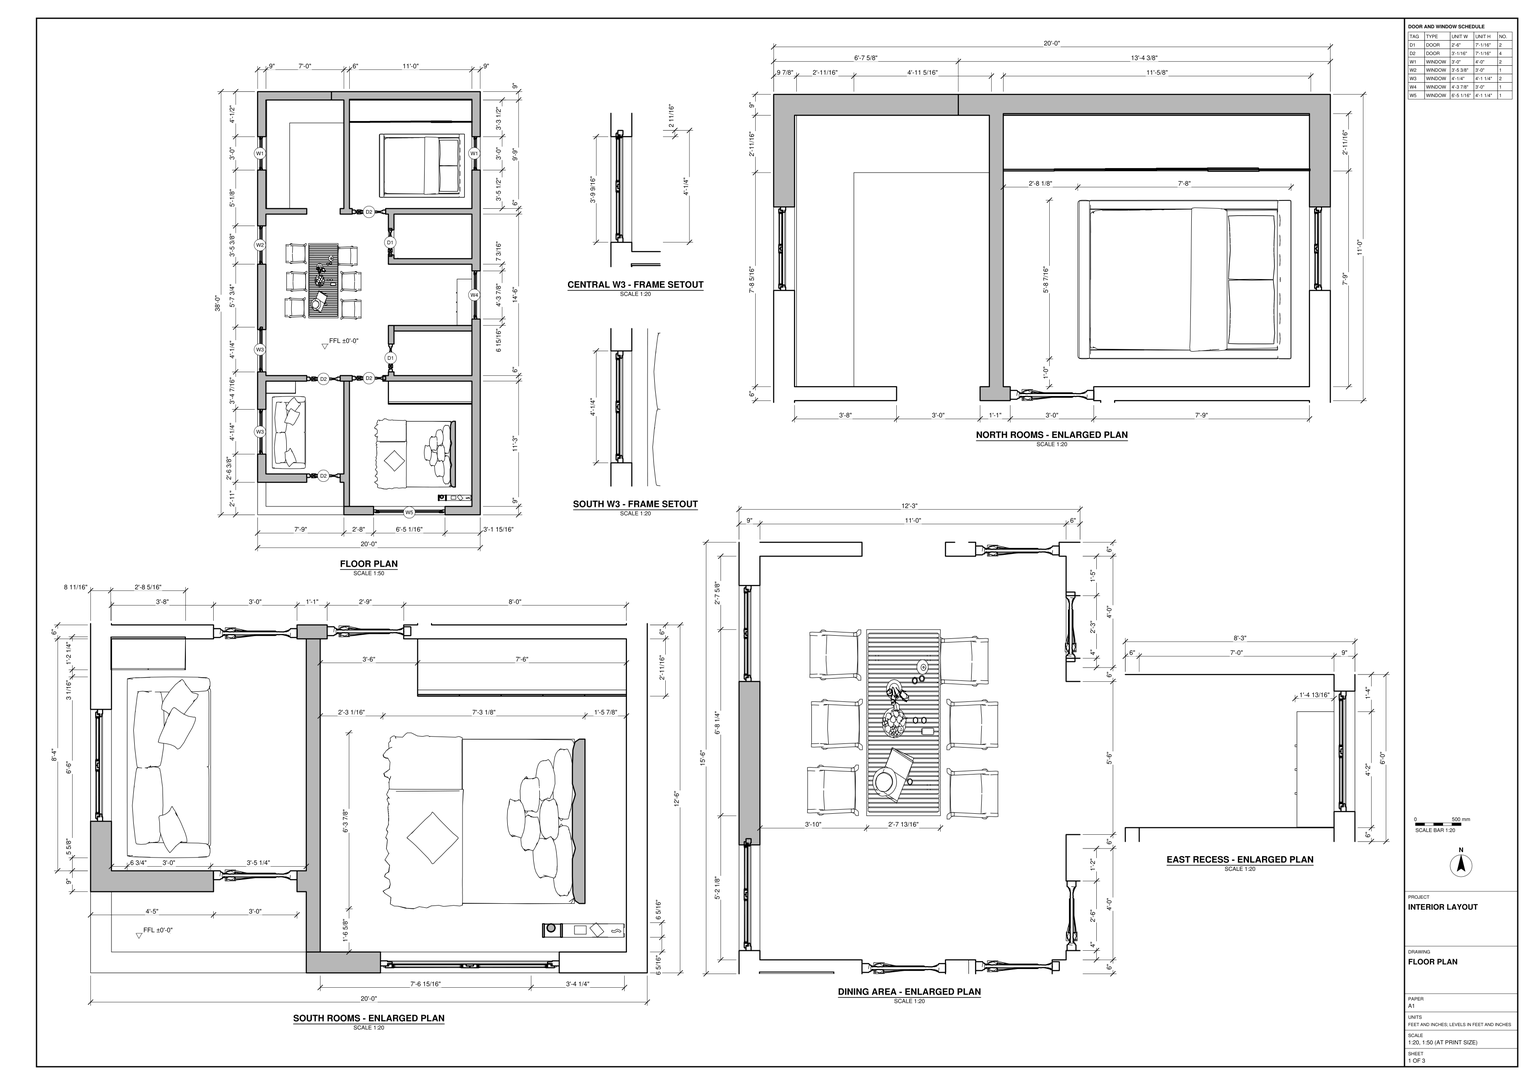
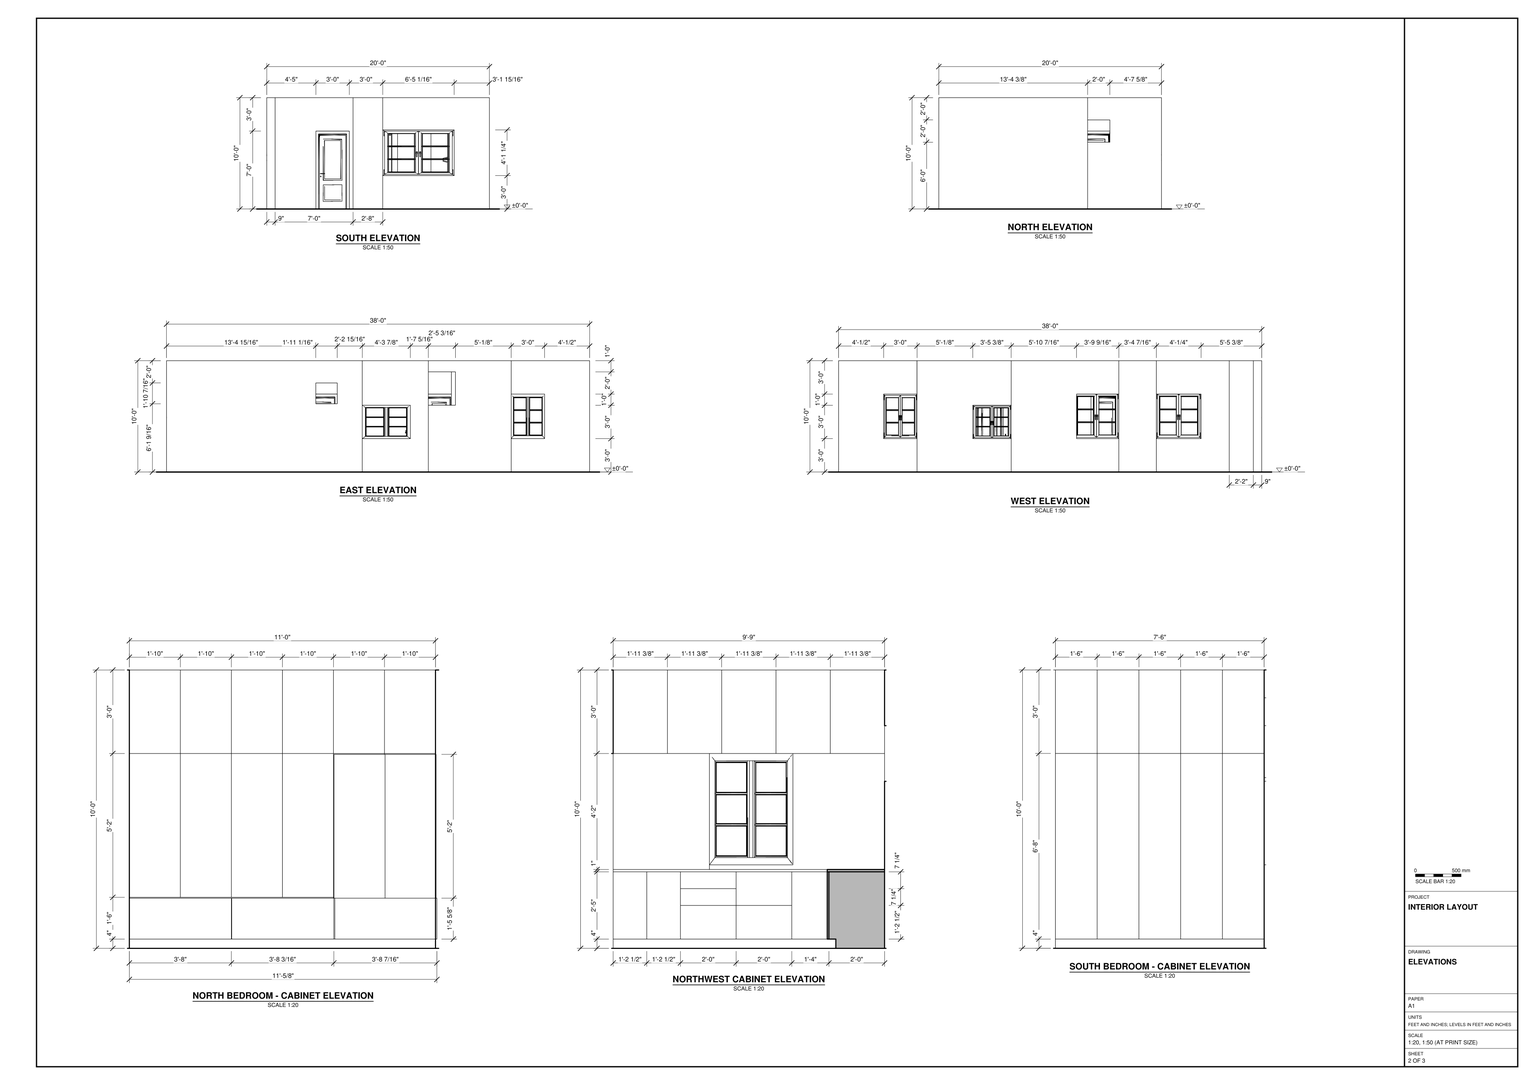
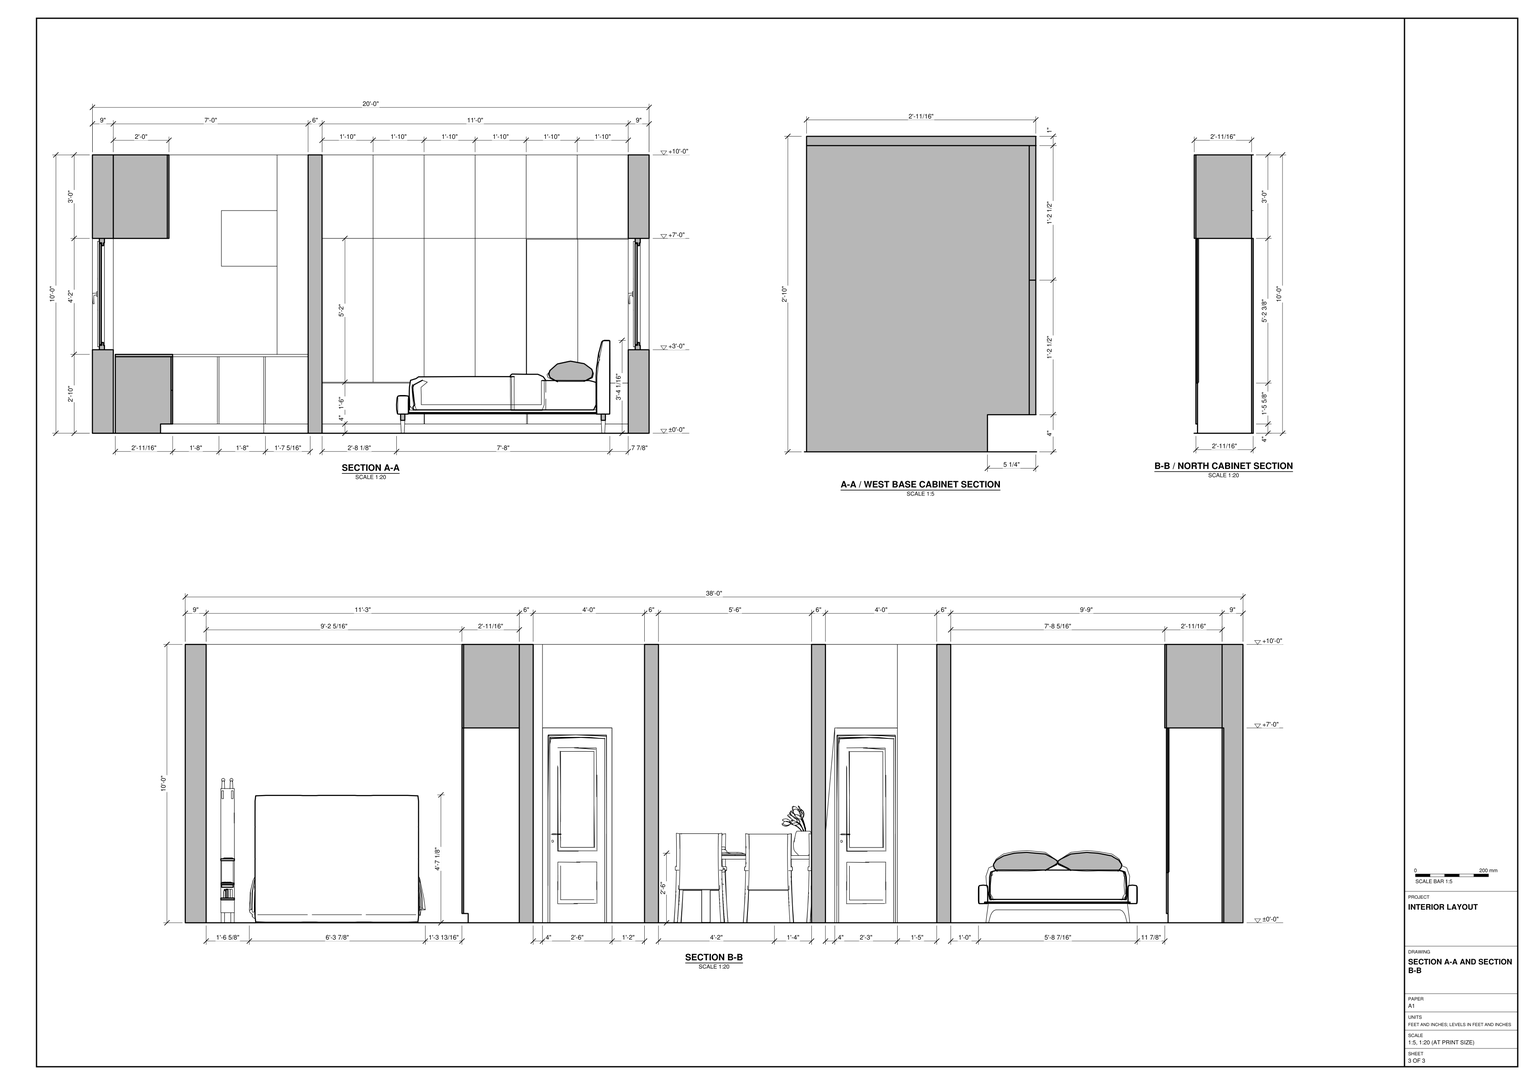
Build the interior in SketchUp from task_files/diagram_01.pdf. Work in feet and inches. The overall model extents are 54'-9 9/16" along X, 65'-5/8" along Y and 10'-13/16" along Z. Use the single finished floor level of ±0'-0". For the room shell itself, follow the 20'-0" by 38'-0" plan and the 10'-0" wall height shown in the sections.

Model the floor slab, the 9" perimeter walls and the 6" partitions, including the setback at the southwest entrance. Lay out the central dining area with its east recess between two enclosed spaces. Use the enlarged plans to position the doors and window units, and the elevations and frame details to set the window heads, sills and divisions.

Place the platform bed in the northeast bedroom, the other bed in the southeast bedroom and the sofa along the west wall of the southwest room. Set the dining table lengthwise with chairs on both long sides. Model the bedroom cabinet runs and the northwest cabinetry around the window, using the cabinet elevations and sections for panel divisions, base units and upper storage. Decor and loose items may be represented by any suitable library components.

Keep shell elements and each furniture or joinery piece in separate groups or components, and use components for repeated parts. Save one SketchUp model as output_files/furnished_two_bedroom_interior_with_built_in_cabinetry.skp.

# SketchUp Ruby script. Lengths in inches.
U = 1.inch
M = Sketchup.active_model
def pt(a) = Geom::Point3d.new(a.map { |v| v * U })
def face(e, loops, mat)
  f = e.add_face(loops[0].map { |a| pt(a) })
  loops[1..].each { |l| e.add_face(l.map { |a| pt(a) }).erase! }
  f.material = f.back_material = mat if mat
  f
end
# faces: each face lists its corners as indices into pts; further lists are holes
def faces(e, pts, list, mat = nil) = list.each { |f| face(e, (f[0].is_a?(Array) ? f : [f]).map { |l| l.map { |i| pts[i] } }, mat) }
# xy, xz, yz: faces in a plane at the given z, y or x. An outline is a flat list of corners, or four numbers for a rectangle; further outlines are holes
def ring(l) = l.size == 4 ? [[l[0], l[1]], [l[2], l[1]], [l[2], l[3]], [l[0], l[3]]] : l.each_slice(2).to_a
def flat(e, list, mat, &to3) = list.each { |f| face(e, (f[0].is_a?(Array) ? f : [f]).map { |l| ring(l).map { |u, v| to3.(u, v) } }, mat) }
def xy(e, z, list, mat = nil) = flat(e, list, mat) { |x, y| [x, y, z] }
def xz(e, y, list, mat = nil) = flat(e, list, mat) { |x, z| [x, y, z] }
def yz(e, x, list, mat = nil) = flat(e, list, mat) { |y, z| [x, y, z] }
def lines(e, pts, list) = list.each { |a, b| e.add_line(pt(pts[a]), pt(pts[b])) }
# prism: a flat outline (further loops are holes) pulled along v
def prism(e, loops, v, mat = nil)
  f = face(e, loops, mat); d = Geom::Vector3d.new(v.map { |x| x * U })
  f.pushpull(f.normal.samedirection?(d) ? d.length : -d.length)
end
def box(e, o, s, mat = nil) = prism(e, [[o, [o[0] + s[0], o[1], o[2]], [o[0] + s[0], o[1] + s[1], o[2]], [o[0], o[1] + s[1], o[2]]]], [0, 0, s[2]], mat)
def at(x, y, z, deg = 0) = Geom::Transformation.translation(pt([x, y, z])) * Geom::Transformation.rotation(ORIGIN, Z_AXIS, deg.degrees)
def axes(o, x, y, z) = Geom::Transformation.new([*x, 0, *y, 0, *z, 0, *pt(o).to_a, 1])
def part(name) = M.definitions.add(name)
# library, detail: a bought-in or finely detailed component or shape, given as its bounding box
def library(name, o, s) = part(name).tap { |d| box(d.entities, o, s) }
def detail(e, o, s) = box(e.add_group.entities, o, s)
def put(e, d, t, mat = nil) = e.add_instance(d, t).tap { |i| i.material = mat if mat }
def group(e, t, mat = nil) = e.add_group.tap { |g| g.transformation = t; g.material = mat if mat }.entities
root = M.entities
M.materials.add("[Basic Tile]").color = [203, 206, 202]
M.materials.add("[Carrera Marble]").color = [207, 207, 207]
M.materials.add("[Color M02]").color = [198, 198, 198]
M.materials.add("[Marble Carrara Gold Floor Tile]").color = [225, 223, 217]
M.materials.add("[Stone Marble]").color = [143, 138, 136]
M.materials.add("[Stone Vein Gray]").color = [166, 165, 165]
M.materials.add("[Wood Bamboo]").color = [177, 105, 43]
M.materials.add("[Wood Board Cork]").color = [215, 201, 115]
M.materials.add("[Wood Lumber ButtJoined]").color = [164, 152, 112]
c1 = library("Tyler Platform Bed",[-34.22,-45.98,0],[68.44,91.98,40.05])
c2 = library("Bed 003",[-38.05,-87.1,0],[75.86,87.1,55.12])
c3 = library("Door 243 074",[-20.11,-2.41,0],[40.22,4.82,86.63])
c4 = library("Dresser 007",[-25,-8.85,0],[50,16.83,30])
c5 = library("Furniture Set 193 001",[-52.77,-40.82,-0.19],[105.38,81.69,50.41])
c6 = library("Giraffe Shelf 96-02",[-20.14,-3.15,0.05],[40.26,6.32,62.23])
c7 = library("Sofa Two-Seater 002",[-38.93,-17.99,0],[77.99,35.98,35.98])
c8 = library("Dresser 002",[-16.14,-8.46,0],[32.28,16.53,40.55])
c9 = library("Window 46-30",[-29.96,-2.6,0],[59.92,5.19,59.84])
c10 = part("Group\#2")
xy(c10.entities,0,[[0,0,22,0.71]])
xy(c10.entities,62,[[0,0,22,0.71]])
xz(c10.entities,0,[[0,0,22,62]],"[Wood Lumber ButtJoined]")
xz(c10.entities,0.71,[[0,0,22,62]])
yz(c10.entities,0,[[0,0,0.71,62]])
yz(c10.entities,22,[[0,0,0.71,62]])
c11 = part("Group\#14")
box(c11.entities,[0,0,0],[22,0.71,62])
c12 = part("Group\#4")
box(c12.entities,[0,0,0],[22,0.71,36])
c13 = part("Group\#9")
box(c13.entities,[0,0,0],[18,0.71,36])
c14 = part("Group\#8")
box(c14.entities,[0,0,0],[18,0.71,80])
c15 = part("Group\#19")
box(c15.entities,[0,-8,0],[0.71,24,14.5])
c16 = part("Group\#17")
box(c16.entities,[0,-8,0],[0.71,24,7.25])
c17 = part("Group\#16")
box(c17.entities,[0.71,0,0],[19.29,0.71,29])
c18 = part("Group\#18")
prism(c18.entities,[[[0,1.5,0],[0,1.5,14.5],[0,1.5,29],[0,16,29],[0,16,0]]],[0.71,0,0])
c19 = part("Group\#22")
box(c19.entities,[0,0,0],[0.71,23.4,36])
xy(root,0,[[[0,0,657.5625,780.625],[20.875,36.8125,260.875,492.8125]],[20.875,36.8125,113.875,36.8125,113.875,45.8125,29.875,45.8125,29.875,71.8125,20.875,71.8125],[113.875,36.8125,145.86,45.8125],[145.86,36.8125,260.875,36.8125,260.875,408.3125,251.875,408.3125,251.875,366.8125,158.875,366.8125,158.875,360.8125,161.875,360.8125,161.875,343.8125,167.875,343.8125,167.875,360.8125,251.875,360.8125,251.875,312.8125,167.875,312.8125,167.875,316.8125,161.875,316.8125,161.875,306.8125,251.875,306.8125,251.875,186.8125,167.875,186.8125,167.875,190.8125,161.875,190.8125,161.875,186.8125,155.875,186.8125,155.875,180.8125,251.875,180.8125,251.875,45.8125,145.86,45.8125],[20.875,71.8125,73.875,71.8125,73.875,80.8125,29.875,80.8125,29.875,180.8125,73.875,180.8125,73.875,186.8125,29.875,186.8125,29.875,360.8125,73.875,360.8125,73.875,366.8125,29.875,366.8125,29.875,483.8125,100.49,483.8125,100.49,492.8125,20.875,492.8125],
  [161.875,156.8125,251.875,180.8125],[109.875,180.8125,119.875,186.8125],[161.875,220.8125,167.875,240.8125],[167.875,234.8125,251.875,240.8125],[161.875,316.8125,167.875,343.8125],
  [109.875,360.8125,122.875,360.8125,122.875,366.8125,119.875,366.8125,119.875,483.8125,251.875,483.8125,251.875,444.3125,260.875,444.3125,260.875,492.8125,100.49,492.8125,100.49,483.8125,113.875,483.8125,113.875,366.8125,109.875,366.8125],[29.875,366.8125,53.875,366.8125,53.875,459.8125,113.875,459.8125,113.875,483.8125,29.875,483.8125],[251.875,408.3125,260.875,444.3125],[119.875,459.8125,251.875,483.8125]])
xy(root,0,[[167.875,312.8125,251.875,360.8125]],"[Stone Marble]")
xy(root,0,[[29.875,45.8125,113.875,45.8125,113.875,71.8125,109.875,71.8125,109.875,80.8125,113.875,80.8125,113.875,180.8125,109.875,180.8125,109.875,186.8125,122.875,186.8125,122.875,180.8125,119.875,180.8125,119.875,45.8125,251.875,45.8125,251.875,156.8125,161.875,156.8125,161.875,180.8125,155.875,180.8125,155.875,186.8125,161.875,186.8125,161.875,190.8125,167.875,190.8125,167.875,186.8125,251.875,186.8125,251.875,234.8125,167.875,234.8125,167.875,220.8125,161.875,220.8125,161.875,240.8125,251.875,240.8125,251.875,306.8125,161.875,306.8125,161.875,360.8125,158.875,360.8125,158.875,366.8125,251.875,366.8125,251.875,459.8125,119.875,459.8125,119.875,366.8125,122.875,366.8125,122.875,360.8125,109.875,360.8125,109.875,366.8125,113.875,366.8125,113.875,459.8125,53.875,459.8125,53.875,366.8125,73.875,366.8125,73.875,360.8125,29.875,360.8125,29.875,186.8125,73.875,186.8125,73.875,180.8125,29.875,180.8125,29.875,80.8125,73.875,80.8125,73.875,71.8125,29.875,71.8125]],"[Stone Vein Gray]")
xy(root,36,[[145.86,36.8125,222.92,45.8125],[20.875,102.16,29.875,150.4],[20.875,190.8125,29.875,236.375],[251.875,247.74,260.875,299.65],[20.875,306.8125,29.875,348.1875],
  [20.875,408.3125,29.875,444.3125]])
xy(root,72,[[251.875,247.74,260.875,299.65],[20.875,306.8125,29.875,348.1875],[251.875,318.98,260.875,348.1875],[76.49,483.8125,100.49,492.8125]])
xy(root,73.59,[[251.875,197.72,260.875,220.8125]])
xy(root,84,[[73.875,71.8125,109.875,80.8125],[20.875,102.16,29.875,150.4],[73.8125,180.8125,109.875,186.8125],[20.875,190.8125,29.875,236.375],[161.875,190.8125,167.875,220.8125],
  [161.875,316.8125,167.875,343.8125],[73.875,360.8125,109.875,366.8125],[29.875,366.8125,53.17,483.8125],[20.875,408.375,29.875,444.3125]])
xy(root,85.26,[[145.86,36.8125,222.92,45.8125]])
xy(root,96,[[251.875,197.72,260.875,220.8125],[76.49,483.8125,100.49,492.8125]])
xy(root,108,[[251.875,318.98,260.875,348.1875]])
xy(root,120,[[113.875,36.8125,145.86,45.8125],[145.86,36.8125,260.875,36.8125,260.875,318.98,251.875,318.98,251.875,45.8125,145.86,45.8125],[113.875,45.8125,119.875,45.8125,119.875,180.8125,113.875,180.8125,113.875,80.8125,29.875,80.8125,29.875,150.4,20.875,150.4,20.875,71.8125,113.875,71.8125],[20.875,150.4,29.875,150.4,29.875,180.8125,73.8125,180.8125,73.8125,186.8125,29.875,186.8125,29.875,190.8125,20.875,190.8125],[73.8125,180.8125,73.875,186.8125],
  [73.875,180.8125,119.875,186.8125],[119.875,180.8125,251.875,180.8125,251.875,186.8125,167.875,186.8125,167.875,240.8125,161.875,240.8125,161.875,186.8125,119.875,186.8125],[20.875,190.8125,29.875,190.8125,29.875,360.8125,109.875,360.8125,109.875,366.8125,29.875,366.8125,29.875,408.3125,20.875,408.3125],[167.875,234.8125,251.875,240.8125],[161.875,306.8125,251.875,306.8125,251.875,312.8125,167.875,312.8125,167.875,343.8125,161.875,343.8125],
  [251.875,318.98,260.875,408.3125],[161.875,343.8125,167.875,343.8125,167.875,360.8125,251.875,360.8125,251.875,366.8125,158.875,366.8125,158.875,360.8125,161.875,360.8125],[29.875,366.8125,53.17,483.8125],[20.875,408.375,29.875,408.375,29.875,483.8125,100.49,483.8125,100.49,492.8125,20.875,492.8125]])
xz(root,36.8125,[[113.875,0,145.86,120],[145.86,0,260.875,0,260.875,120,145.86,120,145.86,85.26,222.92,85.26,222.92,36,145.86,36]])
xz(root,45.8125,[[113.875,0,119.875,120],[119.875,0,145.86,120],[145.86,0,145.86,36,222.92,36,222.92,85.26,145.86,85.26,145.86,120,251.875,120,251.875,0]])
xz(root,71.8125,[[20.875,0,29.875,120],[29.875,0,73.875,0,73.875,84,109.875,84,109.875,0,113.875,0,113.875,120,29.875,120]])
xz(root,80.8125,[[29.875,0,73.875,120],[109.875,0,109.875,84,73.875,84,73.875,120,113.875,120,113.875,0]])
xz(root,102.16,[[20.875,36,29.875,84]])
xz(root,150.4,[[20.875,36,29.875,84]])
xz(root,180.8125,[[29.875,0,73.875,0,73.875,84,73.8125,84,73.8125,120,29.875,120],[109.875,0,113.875,0,113.875,120,73.875,120,73.875,84,109.875,84],[113.875,0,119.875,120],[119.875,0,122.875,85.3125],[155.875,0,251.875,0,251.875,120,119.875,120,119.875,88.11,122.875,88.11,122.875,85.3125,155.875,85.3125],
  [73.8125,84,73.875,120],[119.875,85.3125,122.875,88.11]])
xz(root,186.8125,[[29.875,0,29.875,120,73.8125,120,73.8125,84,73.875,84,73.875,0],[109.875,0,109.875,84,73.875,84,73.875,120,161.875,120,161.875,0,155.875,0,155.875,88.11,122.875,88.11,122.875,0],[167.875,0,251.875,120],[73.8125,84,73.875,120]])
xz(root,190.8125,[[161.875,0,167.875,84],[20.875,36,29.875,84]])
xz(root,197.72,[[251.875,73.59,260.875,96]])
xz(root,220.8125,[[161.875,0,167.875,84],[251.875,73.59,260.875,96]])
xz(root,234.8125,[[167.875,0,251.875,120]])
xz(root,236.375,[[20.875,36,29.875,84]])
xz(root,240.8125,[[161.875,0,167.875,120],[167.875,0,251.875,120]])
xz(root,247.74,[[251.875,36,260.875,72]])
xz(root,299.65,[[251.875,36,260.875,72]])
xz(root,306.8125,[[161.875,0,251.875,120],[20.875,36,29.875,72]])
xz(root,312.8125,[[167.875,0,251.875,120]])
xz(root,316.8125,[[161.875,0,167.875,84]])
xz(root,318.98,[[251.875,72,260.875,108]])
xz(root,343.8125,[[161.875,0,167.875,84]])
xz(root,348.1875,[[20.875,36,29.875,72],[251.875,72,260.875,108]])
xz(root,360.8125,[[29.875,0,73.875,0,73.875,84,109.875,84,109.875,120,29.875,120],[158.875,0,161.875,120],[167.875,0,251.875,120]])
xz(root,366.8125,[[29.875,0,29.875,84,53.17,84,53.17,120,109.875,120,109.875,84,73.875,84,73.875,0],[158.875,0,251.875,120],[29.875,84,53.17,120]])
xz(root,408.3125,[[251.875,0,260.875,120],[20.875,36,29.875,120]])
xz(root,408.375,[[20.875,84,29.875,120]])
xz(root,444.3125,[[20.875,36,29.875,84]])
xz(root,483.8125,[[29.875,0,100.49,0,100.49,72,76.49,72,76.49,96,100.49,96,100.49,120,53.17,120,53.17,84,29.875,84]])
xz(root,492.8125,[[20.875,0,20.875,120,100.49,120,100.49,96,76.49,96,76.49,72,100.49,72,100.49,0]])
yz(root,20.875,[[71.8125,0,71.8125,120,150.4,120,150.4,84,102.16,84,102.16,36,150.4,36,150.4,0],[150.4,0,190.8125,120],[190.8125,0,190.8125,36,236.375,36,236.375,84,190.8125,84,190.8125,120,306.8125,120,306.8125,0],[306.8125,0,306.8125,36,348.1875,36,348.1875,72,306.8125,72,306.8125,120,408.3125,120,408.3125,0],[408.3125,0,408.3125,36,444.3125,36,444.3125,84,408.375,84,408.375,120,492.8125,120,492.8125,0]])
yz(root,29.875,[[80.8125,0,150.4,0,150.4,36,102.16,36,102.16,84,150.4,84,150.4,120,80.8125,120],[150.4,0,180.8125,120],[186.8125,0,190.8125,120],[190.8125,0,306.8125,0,306.8125,72,348.1875,72,348.1875,36,306.8125,36,306.8125,0,360.8125,0,360.8125,120,190.8125,120,190.8125,84,236.375,84,236.375,36,190.8125,36],[366.8125,84,408.3125,120],
  [408.3125,84,408.375,120],[408.375,84,483.8125,120]])
yz(root,29.875,[[366.8125,0,408.3125,84],[408.3125,0,483.8125,0,483.8125,84,444.3125,84,444.3125,36,408.3125,36]],"[Basic Tile]")
yz(root,53.17,[[366.8125,84,390.21,120],[390.21,84,413.61,120],[413.61,84,437.01,120],[437.01,84,460.41,120],[460.41,84,483.8125,120]])
yz(root,73.8125,[[180.8125,84,186.8125,120]])
yz(root,73.875,[[71.8125,0,80.8125,84],[180.8125,0,186.8125,120],[360.8125,0,366.8125,84]])
yz(root,76.49,[[483.8125,72,492.8125,96]])
yz(root,100.49,[[483.8125,0,492.8125,72],[483.8125,96,492.8125,120]])
yz(root,109.875,[[71.8125,0,80.8125,84],[180.8125,0,186.8125,84],[360.8125,84,366.8125,120]])
yz(root,113.875,[[36.8125,0,45.8125,120],[45.8125,0,71.8125,120],[80.8125,0,180.8125,120]])
yz(root,119.875,[[45.8125,0,180.8125,120],[180.8125,85.3125,180.8125,88.11,186.8125,88.11]])
yz(root,122.875,[[180.8125,0,186.8125,88.11]])
yz(root,145.86,[[36.8125,36,45.8125,85.26]])
yz(root,155.875,[[180.8125,0,180.8125,85.3125,186.8125,88.11,186.8125,0]])
yz(root,158.875,[[360.8125,0,366.8125,120]])
yz(root,161.875,[[186.8125,0,186.8125,120,240.8125,120,240.8125,0,220.8125,0,220.8125,84,190.8125,84,190.8125,0],[306.8125,0,306.8125,120,360.8125,120,360.8125,0,343.8125,0,343.8125,84,316.8125,84,316.8125,0]])
yz(root,167.875,[[186.8125,0,190.8125,120],[220.8125,0,234.8125,0,234.8125,120,190.8125,120,190.8125,84,220.8125,84],[234.8125,0,240.8125,120],[312.8125,0,316.8125,0,316.8125,84,343.8125,84,343.8125,120,312.8125,120],[343.8125,0,360.8125,120]])
yz(root,222.92,[[36.8125,36,45.8125,85.26]])
yz(root,251.875,[[45.8125,0,180.8125,120],[186.8125,0,197.72,120],[197.72,0,197.72,73.59,220.8125,73.59,220.8125,96,197.72,96,197.72,120,234.8125,120,234.8125,0],[234.8125,0,240.8125,120],[[240.8125,0,306.8125,120],[247.74,36,299.65,72]],
  [312.8125,0,318.98,120],[318.98,0,318.98,72,348.1875,72,348.1875,108,318.98,108,318.98,120,360.8125,120,360.8125,0],[366.8125,0,408.3125,120]])
yz(root,260.875,[[[36.8125,0,247.74,120],[197.72,73.59,220.8125,96]],[247.74,0,318.98,0,318.98,120,247.74,120,247.74,72,299.65,72,299.65,36,247.74,36],[318.98,0,408.3125,0,408.3125,120,318.98,120,318.98,108,348.1875,108,348.1875,72,318.98,72]])
p = [[176.95,309.46,0],[167.875,316.8125,84]]
lines(root,p,[[0,1]])
put(root,c1,at(197.97,413,0,-90))
put(root,c2,at(234.02,102.24,0,-90))
put(root,c3,axes([91.84,78.83,-0.07],[0.89652,0,0],[0,1,0],[0,0,0.97036]),"[Wood Bamboo]")
put(root,c3,axes([91.91,183.22,0],[0.89652,0,0],[0,1,0],[0,0,0.97036]),"[Wood Bamboo]")
put(root,c3,axes([140.91,363.22,0],[0.89652,0,0],[0,1,0],[0,0,0.97036]),"[Wood Bamboo]")
put(root,c3,axes([140.91,184.03,0],[0.89652,0,0],[0,1,0],[0,0,0.97036]),"[Wood Bamboo]")
put(root,c3,axes([164.28,205.8125,0],[0,0.74575,0],[-1,0,0],[0,0,0.97036]),"[Wood Bamboo]")
put(root,c4,at(243.89,265.8125,0,-90))
put(root,c5,axes([91.51,288.31,0.19],[0.78,0,0],[0,1,0],[0,0,1]))
put(root,c6,at(230.93,55.3,0))
put(root,c7,at(54.65,125.36,0,90))
put(root,c8,axes([45.7,174.74,-0.8],[1,0,0],[0,0.86,0],[0,0,0.66]))
put(root,c9,axes([184.39,39.41,36],[1.28607,0,0],[0,1,0],[0,0,0.82314]))
put(root,c9,axes([23.47,126.28,36],[0,-0.805,0],[1,0,0],[0,0,0.82314]))
put(root,c9,axes([23.47,214.93,36],[0,-0.805,0],[1,0,0],[0,0,0.82314]))
put(root,c9,axes([23.47,327.5,36],[0,-0.69053,0],[1,0,0],[0,0,0.60162]))
put(root,c9,axes([23.47,426.3125,36],[0,-0.60083,0],[1,0,0],[0,0,0.80216]))
put(root,c9,axes([254.47,426.3125,36],[0,-0.60083,0],[1,0,0],[0,0,0.80216]))
put(root,c9,axes([254.47,273.7,36],[0,-0.86627,0],[1,0,0],[0,0,0.60162]))
put(root,c3,axes([163.86,330.36,-0.0625],[0,0.74575,0],[-1,0,0],[0,0,0.97036]),"[Wood Bamboo]")
g1 = group(root,at(100.49,360.8125,0))
xy(g1,0,[[9.38,0,9.38,6,13.38,6,13.38,123,0,123,0,132,160.38,132,160.38,47.5,151.38,47.5,151.38,123,19.38,123,19.38,6,22.38,6,22.38,0]])
xy(g1,36,[[151.38,47.5,160.38,83.5]])
xy(g1,84,[[22.38,0,58.38,6],[151.38,47.5,160.38,83.5]])
xy(g1,120,[[9.38,0,58.38,0,58.38,6,19.38,6,19.38,123,151.38,123,151.38,47.5,160.38,47.5,160.38,132,0,132,0,123,13.38,123,13.38,6,9.38,6]])
xz(g1,0,[[9.38,0,22.38,0,22.38,84,58.38,84,58.38,120,9.38,120]])
xz(g1,6,[[9.38,0,13.38,120],[19.38,0,19.38,120,58.38,120,58.38,84,22.38,84,22.38,0]])
xz(g1,47.5,[[151.38,0,160.38,36],[151.38,84,160.38,120]])
xz(g1,83.5,[[151.38,36,160.38,84]])
xz(g1,123,[[0,0,13.38,120],[19.38,0,151.38,120]])
xz(g1,132,[[0,0,160.38,120]])
yz(g1,0,[[123,0,132,120]])
yz(g1,9.38,[[0,0,6,120]])
yz(g1,13.38,[[6,0,123,120]])
yz(g1,19.38,[[6,0,123,120]])
yz(g1,22.38,[[0,0,6,84]])
yz(g1,58.38,[[0,84,6,120]])
yz(g1,151.38,[[47.5,0,47.5,36,83.5,36,83.5,84,47.5,84,47.5,120,123,120,123,0]])
yz(g1,160.38,[[47.5,0,132,0,132,120,47.5,120,47.5,84,83.5,84,83.5,36,47.5,36]])
put(root,c10,at(230.12,459.96,21.62),"[Color M02]")
g2 = group(root,at(119.875,459.8125,0),"[Wood Lumber ButtJoined]")
xy(g2,0,[[0,0.71,132,24.71]],"[Wood Lumber ButtJoined]")
xy(g2,84,[[0,0.71,132,24.71]],"[Wood Lumber ButtJoined]")
xz(g2,0.71,[[0,0,132,4],[0,4,44,21.62],[44,4,88,4,88,22,0,22,0,21.62,44,21.62],[88,4,132,22],[0,22,22,84],
  [22,22,44,84],[44,22,66,84],[66,22,88,84],[88,22,110,84],[110,22,132,84]],"[Wood Lumber ButtJoined]")
xz(g2,24.71,[[0,0,132,84]],"[Wood Lumber ButtJoined]")
yz(g2,0,[[0.71,0,24.71,84]],"[Wood Lumber ButtJoined]")
yz(g2,132,[[0.71,0,24.71,84]],"[Wood Lumber ButtJoined]")
put(g2,c11,at(88,0.57,22),"[Color M02]")
put(g2,c11,at(0,0,22),"[Wood Lumber ButtJoined]")
put(g2,c11,at(22,0.14,22),"[Wood Lumber ButtJoined]")
put(g2,c11,at(44,0.28,22),"[Wood Lumber ButtJoined]")
put(g2,c11,at(66,0.43,22),"[Wood Lumber ButtJoined]")
g3 = group(g2,at(0,0,4),"[Color M02]")
prism(g3,[[[44,0,0],[44,0,17.62],[22,0,17.62],[0,0,17.62],[0,0,0]]],[0,0.71,0],"[Wood Lumber ButtJoined]")
g4 = group(g2,at(44.16,0,4),"[Wood Lumber ButtJoined]")
prism(g4,[[[44,0,0],[44,0,17.62],[22,0,17.62],[0,0,17.62],[0,0,0]]],[0,0.71,0],"[Wood Lumber ButtJoined]")
g5 = group(g2,at(88.59,0,4),"[Wood Lumber ButtJoined]")
prism(g5,[[[44,0,0],[44,0,17.62],[22,0,17.62],[0,0,17.62],[0,0,0]]],[0,0.71,0],"[Wood Lumber ButtJoined]")
g6 = group(root,at(119.875,459.1,84),"[Wood Lumber ButtJoined]")
put(g6,c12,at(110,0,0))
g7 = group(g6,at(0,0,0))
xy(g7,0,[[0,0.71,132,24.71]])
xy(g7,36,[[0,0.71,132,24.71]])
xz(g7,0.71,[[0,0,110,36],[110,0,132,36]])
xz(g7,24.71,[[0,0,132,36]])
yz(g7,0,[[0.71,0,24.71,36]])
yz(g7,132,[[0.71,0,24.71,36]])
put(g7,c12,at(88,0,0))
put(g7,c12,at(66,0,0))
put(g7,c12,at(44,0,0))
put(g7,c12,at(0,0,0))
put(g7,c12,at(22,0,0))
g8 = group(root,at(251.875,180.8125,84,-180),"[Wood Board Cork]")
xy(g8,0,[[0,0,90,24]])
xy(g8,36,[[0,0,90,24]])
xz(g8,0,[[0,0,90,36]])
xz(g8,24,[[0,0,18,36],[18,0,90,36]])
yz(g8,0,[[0,0,24,36]])
yz(g8,90,[[0,0,24,36]])
put(g8,c13,at(54,24,0))
put(g8,c13,at(72,24,0))
put(g8,c13,at(36,24,0))
put(g8,c13,at(0,24,0))
put(g8,c13,at(18,24,0))
g9 = group(root,at(251.875,180.8125,0,-180),"[Wood Board Cork]")
xy(g9,0,[[0,0,90,22.03]])
xy(g9,4,[[0,22.03,90,24]])
xy(g9,84,[[0,0,90,24]])
xz(g9,0,[[0,0,90,84]])
xz(g9,22.03,[[0,0,90,4]])
xz(g9,24,[[0,4,18,84],[18,4,90,84]])
yz(g9,0,[[0,0,0,84,24,84,24,4,22.03,4,22.03,0]])
yz(g9,90,[[0,0,22.03,0,22.03,4,24,4,24,84,0,84]])
put(g9,c14,at(18,24,4))
put(g9,c14,at(72,24,4))
put(g9,c14,at(54,24,4))
put(g9,c14,at(0,24,4))
put(g9,c14,at(36,24,4))
put(root,c10,at(208.12,459.68,21.62),"[Color M02]")
g10 = group(root,at(30.75,366.8125,0))
xy(g10,0,[[0,0,0,117,84,117,84,96,19.5,96,19.5,0]])
xy(g10,4,[[19.5,0,24,96],[24,93,64,96],[64,93,84,96]])
xy(g10,33,[[0,0,24,0,24,93,84,93,84,117,0,117]])
xz(g10,0,[[0,0,19.5,0,19.5,4,24,4,24,33,0,33]])
xz(g10,93,[[24,4,44,33],[44,4,64,33],[64,4,84,33]])
xz(g10,96,[[19.5,0,64,4],[64,0,84,4]])
xz(g10,117,[[0,0,70.62,33],[70.62,0,84,33]])
yz(g10,0,[[0,0,41.5,33],[41.5,0,117,33]])
yz(g10,19.5,[[0,0,96,4]])
yz(g10,24,[[0,4,14.5,33],[14.5,4,29,33],[29,4,53,18.5],[53,4,77,18.5],[77,4,93,33],
  [29,18.5,53,33],[53,18.5,77,33]])
yz(g10,84,[[96,0,117,0,117,33,93,33,93,4,96,4]])
g11 = group(g10,at(24,77,4))
prism(g11,[[[0,0,14.5],[0,0,29],[0,16,29],[0,16,0],[0,0,0]]],[0.71,0,0])
g12 = group(g10,at(0,0,33),"[Marble Carrara Gold Floor Tile]")
prism(g12,[[[24.71,92.29,0],[24.71,0,0],[0,0,0],[0,41.5,0],[0,117,0],[70.62,117,0],[84,117,0],[84,92.29,0]]],[0,0,1],"[Carrera Marble]")
put(g10,c15,at(24,61,4))
put(g10,c16,at(24,37,18.5))
put(g10,c17,at(64,92.29,4))
put(g10,c15,at(24,61,18.5))
put(g10,c15,at(24,37,4))
put(g10,c17,at(24,92.29,4))
put(g10,c16,at(24,37,25.75))
put(g10,c18,at(24,13,4))
put(g10,c17,at(44,92.29,4))
put(g10,c18,at(24,-1.5,4))
put(root,c19,at(53.17,366.8125,84))
put(root,c19,at(53.17,390.21,84))
put(root,c19,at(53.17,413.61,84))
put(root,c19,at(53.17,437.01,84))
put(root,c19,at(53.17,460.41,84))
